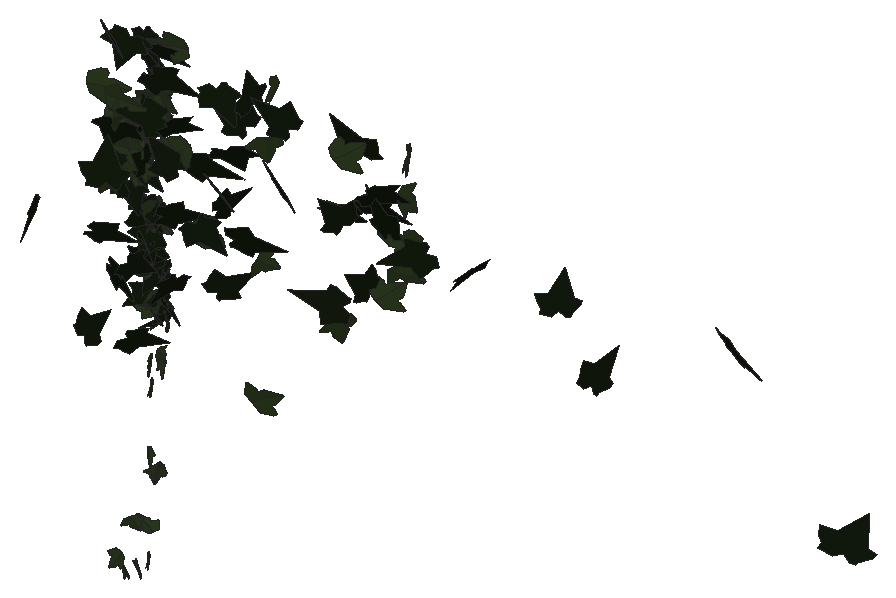
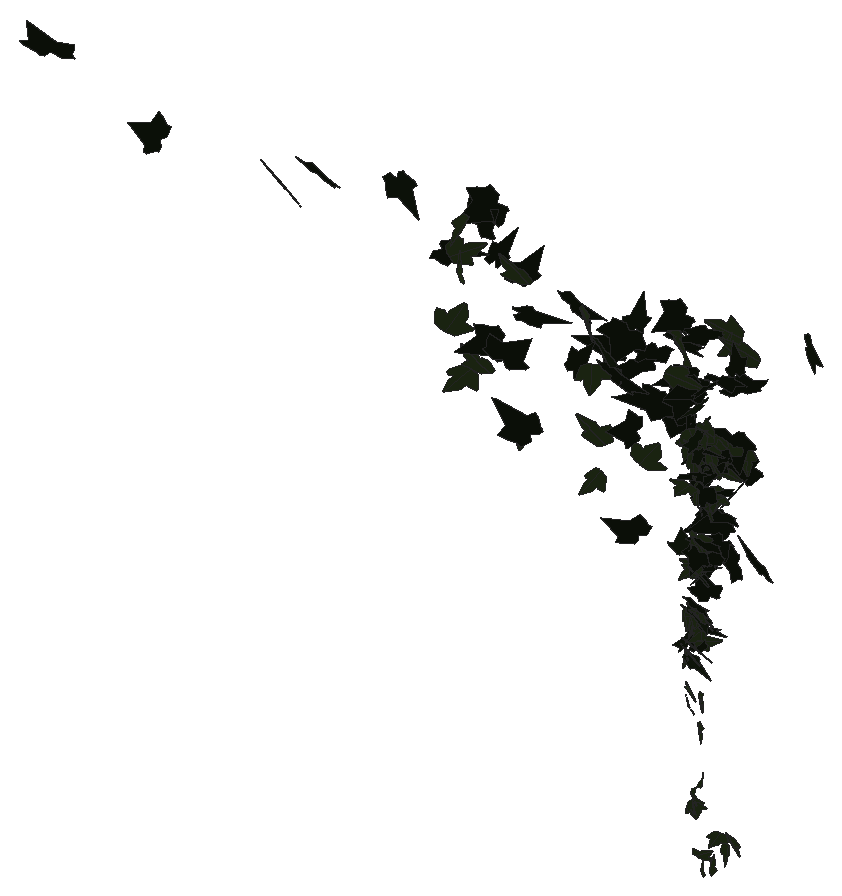
# SketchUp Ruby script. Lengths in inches.
U = 1.inch
M = Sketchup.active_model
def pt(a) = Geom::Point3d.new(a.map { |v| v * U })
def face(e, loops, mat)
  f = e.add_face(loops[0].map { |a| pt(a) })
  loops[1..].each { |l| e.add_face(l.map { |a| pt(a) }).erase! }
  f.material = f.back_material = mat if mat
  f
end
# faces: each face lists its corners as indices into pts; further lists are holes
def faces(e, pts, list, mat = nil) = list.each { |f| face(e, (f[0].is_a?(Array) ? f : [f]).map { |l| l.map { |i| pts[i] } }, mat) }
# xy, xz, yz: faces in a plane at the given z, y or x. An outline is a flat list of corners, or four numbers for a rectangle; further outlines are holes
def ring(l) = l.size == 4 ? [[l[0], l[1]], [l[2], l[1]], [l[2], l[3]], [l[0], l[3]]] : l.each_slice(2).to_a
def flat(e, list, mat, &to3) = list.each { |f| face(e, (f[0].is_a?(Array) ? f : [f]).map { |l| ring(l).map { |u, v| to3.(u, v) } }, mat) }
def xy(e, z, list, mat = nil) = flat(e, list, mat) { |x, y| [x, y, z] }
def xz(e, y, list, mat = nil) = flat(e, list, mat) { |x, z| [x, y, z] }
def yz(e, x, list, mat = nil) = flat(e, list, mat) { |y, z| [x, y, z] }
def lines(e, pts, list) = list.each { |a, b| e.add_line(pt(pts[a]), pt(pts[b])) }
# prism: a flat outline (further loops are holes) pulled along v
def prism(e, loops, v, mat = nil)
  f = face(e, loops, mat); d = Geom::Vector3d.new(v.map { |x| x * U })
  f.pushpull(f.normal.samedirection?(d) ? d.length : -d.length)
end
def box(e, o, s, mat = nil) = prism(e, [[o, [o[0] + s[0], o[1], o[2]], [o[0] + s[0], o[1] + s[1], o[2]], [o[0], o[1] + s[1], o[2]]]], [0, 0, s[2]], mat)
def at(x, y, z, deg = 0) = Geom::Transformation.translation(pt([x, y, z])) * Geom::Transformation.rotation(ORIGIN, Z_AXIS, deg.degrees)
def axes(o, x, y, z) = Geom::Transformation.new([*x, 0, *y, 0, *z, 0, *pt(o).to_a, 1])
def part(name) = M.definitions.add(name)
# library, detail: a bought-in or finely detailed component or shape, given as its bounding box
def library(name, o, s) = part(name).tap { |d| box(d.entities, o, s) }
def detail(e, o, s) = box(e.add_group.entities, o, s)
def put(e, d, t, mat = nil) = e.add_instance(d, t).tap { |i| i.material = mat if mat }
def group(e, t, mat = nil) = e.add_group.tap { |g| g.transformation = t; g.material = mat if mat }.entities
root = M.entities
M.materials.add("1026 AP 7946 SUNNY SIDE UP").color = [254, 231, 186]
M.materials.add("efeu1").color = [18, 25, 13]
M.materials.add("efeu2").color = [43, 57, 29]
c1 = part("ivyleaf_9")
p = [[1.54,2.16,1.25],[1.36,2.04,1.19],[-0.21,0.99,0.68],[-0.71,1.11,0.82],[-0.85,0.86,0.67],[-0.8,0.17,0.21],
  [-0.9,-0.01,0.1],[-0.67,-0.16,-0.02],[-0.08,-0.08,-0.05],[-0.03,-0.6,-0.4],[0.65,-0.88,-0.66],[0.83,-0.6,-0.49],
  [1.29,-0.42,-0.43],[1.8125,-0.07,-0.26],[1.21,0.44,0.15]]
faces(c1.entities,p,[[0,1,2,3,4,5,6,7,8,9,10,11,12,13,14]],"efeu1")
c2 = part("ivyleaf_10")
p = [[0,0.5,-0.03],[-0.0625,2.02,-0.43],[-0.19,2.01,-0.46],[-0.54,1.05,-0.29],[-0.52,0.625,-0.18],[-0.83,0.76,-0.28],
  [-1.16,0.64,-0.33],[-1.15,0.33,-0.24],[-0.77,-0.39,0.02],[-0.3,-0.51,0.16],[0.04,-0.48,0.23],[-0.02,2.01,-0.4375],
  [-0.06,2.01,-0.43],[0.04,-0.49,0.23],[0.67,-0.49,0.14],[1.38,0.36,-0.2],[1.375,0.51,-0.24],[0.81,0.65,-0.19],
  [0.62,0.59,-0.15],[0.6,1.09,-0.28],[0.5,1.23,-0.31]]
faces(c2.entities,p,[[0,1,2,3,4,5,6,7,8,9,10],[11,12,0,13,14,15,16,17,18,19,20]],"efeu2")
put(root,c1,axes([145.81,210.97,267.7],[-0.10226,-0.06705,0.33732],[0.10741,-0.32957,-0.05741],[0.51504,0.05542,0.07895]),"1026 AP 7946 SUNNY SIDE UP")
put(root,c2,axes([145.85,211.23,264.91],[0.40959,0.12772,-0.13372],[0.15878,0.08873,0.29755],[0.23926,-0.27752,0.03146]),"1026 AP 7946 SUNNY SIDE UP")
put(root,c2,axes([145.9375,211.7,251.53],[-0.19651,-0.13875,-0.10808],[0.14363,0.05646,-0.19013],[0.23189,-0.15255,0.02617]),"1026 AP 7946 SUNNY SIDE UP")
put(root,c1,axes([146.02,211.48,267.62],[-0.40394,-0.18707,-0.07784],[0.12417,0.01748,-0.32567],[0.29125,-0.2669,0.03089]),"1026 AP 7946 SUNNY SIDE UP")
put(root,c2,axes([146.15,212.33,251.04],[0.20297,0.0955,0.12839],[-0.19011,-0.0414,0.16215],[0.15645,-0.1742,0.03047]),"1026 AP 7946 SUNNY SIDE UP")
put(root,c2,axes([145.93,211.33,264.74],[-0.2012,0.25885,-0.12828],[0.08265,-0.11455,-0.29812],[-0.44507,-0.13829,0.00263]),"1026 AP 7946 SUNNY SIDE UP")
put(root,c2,axes([146.16,212.125,263.7],[-0.29001,-0.20187,0.08916],[-0.07666,-0.07409,-0.2818],[0.33749,-0.19031,0.01261]),"1026 AP 7946 SUNNY SIDE UP")
put(root,c2,axes([146.06,212.47,255.6875],[0.11639,-0.22167,-0.06838],[0.0122,0.07073,-0.23852],[0.36308,0.06868,0.02994]),"1026 AP 7946 SUNNY SIDE UP")
put(root,c1,axes([146.16,210.73,265.14],[0.34508,0.18415,-0.24138],[-0.24927,-0.17578,-0.29501],[-0.39831,0.26955,-0.0245]),"1026 AP 7946 SUNNY SIDE UP")
put(root,c1,axes([146.24,212.32,259.63],[-0.00974,0.25184,0.10049],[-0.11375,0.09106,-0.25007],[-0.4083,-0.03138,0.06727]),"1026 AP 7946 SUNNY SIDE UP")
put(root,c2,axes([146.1,212.53,259.7],[-0.35282,0.07848,0.00293],[-0.01517,-0.02036,-0.24391],[-0.12252,-0.22347,0.02177]),"1026 AP 7946 SUNNY SIDE UP")
put(root,c1,axes([146.14,211.09,262.98],[0.05251,-0.30731,-0.04227],[0.07696,-0.03379,0.31492],[-0.48103,-0.03895,0.04577]),"1026 AP 7946 SUNNY SIDE UP")
put(root,c2,axes([146.36,212.11,258.46],[-0.07709,-0.03468,-0.25525],[-0.37568,-0.06776,0.05812],[-0.1157,0.24312,-0.01865]),"1026 AP 7946 SUNNY SIDE UP")
put(root,c1,axes([145.99,212.43,261.75],[-0.06164,-0.24192,0.10022],[0.00245,-0.09998,-0.25251],[0.41081,-0.0357,0.01654]),"1026 AP 7946 SUNNY SIDE UP")
put(root,c1,axes([146.27,212.13,258.95],[-0.35397,-0.09187,0.08629],[-0.0999,-0.06514,-0.24835],[0.16867,-0.23138,0.03399]),"1026 AP 7946 SUNNY SIDE UP")
put(root,c2,axes([146.28,211.89,263.28],[0.11779,-0.11836,-0.26964],[-0.19717,0.22912,-0.14273],[0.4053,0.14585,0.00893]),"1026 AP 7946 SUNNY SIDE UP")
put(root,c2,axes([146.47,211.17,264.22],[0.13088,-0.03505,-0.33312],[-0.48796,0.09069,-0.09194],[0.15208,0.32114,-0.00834]),"1026 AP 7946 SUNNY SIDE UP")
put(root,c2,axes([146.18,211.76,265.04],[-0.0151,-0.29421,-0.00994],[0.00696,0.00784,-0.30318],[0.46274,-0.00972,0.00424]),"1026 AP 7946 SUNNY SIDE UP")
put(root,c1,axes([146.1,212.47,261.8],[0.37145,0.02124,-0.11874],[-0.17629,-0.0355,-0.24343],[-0.05431,0.26049,-0.02193]),"1026 AP 7946 SUNNY SIDE UP")
put(root,c1,axes([145.97,211.9,261.23],[-0.02565,-0.03067,0.28127],[0.38159,0.12698,0.03036],[-0.20311,0.24244,0.02151]),"1026 AP 7946 SUNNY SIDE UP")
put(root,c1,axes([145.98,211.65,263.65],[-0.03308,-0.26621,-0.14639],[0.07427,0.13626,-0.27231],[0.46752,-0.04048,0.0329]),"1026 AP 7946 SUNNY SIDE UP")
put(root,c2,axes([146.125,212.34,256.61],[0.15836,-0.22215,0.0476],[0.08028,-0.02846,-0.24898],[0.34806,0.10764,0.03577]),"1026 AP 7946 SUNNY SIDE UP")
put(root,c2,axes([146.14,212.28,265.875],[-0.34523,0.18958,-0.04181],[0.03447,-0.03828,-0.29869],[-0.30325,-0.22017,0.01364]),"1026 AP 7946 SUNNY SIDE UP")
put(root,c2,axes([146.21,212.57,252.85],[-0.20183,-0.157,0.04092],[0.01719,-0.06006,-0.20392],[0.25441,-0.12049,0.04624]),"1026 AP 7946 SUNNY SIDE UP")
put(root,c1,axes([145.97,212.49,265.4375],[0.33064,-0.18142,-0.01898],[-0.03977,-0.00275,-0.28548],[0.2838,0.21097,-0.01789]),"1026 AP 7946 SUNNY SIDE UP")
put(root,c2,axes([146.21,212.48,259.74],[0.26669,0.12797,-0.11203],[-0.11548,-0.08361,-0.2184],[-0.23829,0.18374,-0.01954]),"1026 AP 7946 SUNNY SIDE UP")
put(root,c2,axes([146.26,210.68,250.87],[0.29654,-0.1606,-0.07067],[-0.09168,0.03584,-0.25476],[0.25825,0.19714,-0.0093]),"1026 AP 7946 SUNNY SIDE UP")
put(root,c2,axes([146.23,211.51,264.84],[0.026,-0.23926,0.21925],[0.04147,-0.21273,-0.24816],[0.50323,0.02989,0.00912]),"1026 AP 7946 SUNNY SIDE UP")
put(root,c1,axes([146.05,212.01,260.18],[0.41203,0.05303,0.03617],[-0.06902,0.04477,0.27039],[0.07201,-0.26052,0.0522]),"1026 AP 7946 SUNNY SIDE UP")
put(root,c2,axes([146.24,212.57,252.97],[-0.10343,-0.19468,0.04011],[0.03786,-0.04967,-0.20834],[0.31022,-0.05885,0.0388]),"1026 AP 7946 SUNNY SIDE UP")
put(root,c1,axes([146.22,211.56,264.72],[0.23555,0.27996,0.02759],[0.03856,0.01542,-0.32668],[-0.4403,0.15112,-0.01385]),"1026 AP 7946 SUNNY SIDE UP")
put(root,c1,axes([146.24,212.25,260.875],[-0.26603,0.20692,-0.00281],[0.01116,0.01084,0.27512],[0.32523,0.16888,-0.01174]),"1026 AP 7946 SUNNY SIDE UP")
put(root,c1,axes([146.09,212.63,260.08],[-0.21443,-0.07293,-0.20014],[0.31084,0.02342,-0.1522],[0.09717,-0.23586,0.04524]),"1026 AP 7946 SUNNY SIDE UP")
put(root,c2,axes([146.24,211.59,263.54],[-0.13151,-0.30108,0.04679],[0.07258,-0.06083,-0.31626],[0.47365,-0.07427,0.06145]),"1026 AP 7946 SUNNY SIDE UP")
put(root,c1,axes([145.97,212.29,263.66],[-0.06827,-0.05391,0.27885],[0.29211,-0.20874,-0.01334],[0.32157,0.17817,0.07132]),"1026 AP 7946 SUNNY SIDE UP")
put(root,c1,axes([146.26,212.7,264.64],[-0.27548,-0.20601,0.02906],[-0.00375,-0.03641,-0.27792],[0.32719,-0.17387,0.02128]),"1026 AP 7946 SUNNY SIDE UP")
put(root,c1,axes([146.4375,212.47,258.01],[-0.23352,0.1948,-0.06346],[-0.01165,-0.08255,-0.24658],[-0.32158,-0.13847,0.05502]),"1026 AP 7946 SUNNY SIDE UP")
put(root,c1,axes([146.05,211.46,262.83],[-0.23725,-0.14339,-0.22558],[0.33357,0.07952,-0.20453],[0.23925,-0.25305,0.06146]),"1026 AP 7946 SUNNY SIDE UP")
put(root,c2,axes([146.09,212.5,263.61],[0.16217,-0.14058,0.21384],[0.22247,-0.15369,-0.17986],[0.32667,0.17445,0.01633]),"1026 AP 7946 SUNNY SIDE UP")
put(root,c2,axes([146.2,212.2,253.66],[-0.04298,0.20191,-0.10179],[0.00806,-0.10011,-0.21034],[-0.35416,-0.02678,0.00756]),"1026 AP 7946 SUNNY SIDE UP")
put(root,c1,axes([146.29,212.375,259.54],[-0.35994,-0.03623,-0.10592],[0.16742,-0.02522,-0.23567],[0.03533,-0.24958,0.03769]),"1026 AP 7946 SUNNY SIDE UP")
put(root,c1,axes([146.51,212.53,258.57],[-0.33225,0.12136,0.05052],[-0.07858,0.00986,-0.25043],[-0.18979,-0.21654,0.01524]),"1026 AP 7946 SUNNY SIDE UP")
put(root,c1,axes([146.1,212.1,267.53],[0.09089,-0.27667,-0.0949],[-0.02992,0.08853,-0.29065],[0.45676,0.06085,-0.00016]),"1026 AP 7946 SUNNY SIDE UP")
put(root,c1,axes([146.13,211.97,263.15],[0.12962,-0.1777,-0.21915],[-0.09651,0.20364,-0.19952],[0.42377,0.10073,0.02159]),"1026 AP 7946 SUNNY SIDE UP")
put(root,c2,axes([146.35,210.8,250.53],[-0.25275,0.17417,0.09181],[-0.11619,0.05137,-0.24314],[-0.28409,-0.17597,0.01776]),"1026 AP 7946 SUNNY SIDE UP")
put(root,c2,axes([146.32,212.46,265.06],[-0.0516,-0.27743,-0.06899],[0.01177,0.06496,-0.28742],[0.44803,-0.03366,-0.00039]),"1026 AP 7946 SUNNY SIDE UP")
put(root,c1,axes([146.05,212.61,265.85],[0.23516,-0.22985,0.06593],[0.03983,-0.06136,-0.2826],[0.37361,0.15122,-0.01137]),"1026 AP 7946 SUNNY SIDE UP")
put(root,c2,axes([146.16,211.87,263.57],[-0.24678,0.14556,-0.20685],[0.17209,-0.17365,-0.21794],[-0.3511,-0.18742,0.03857]),"1026 AP 7946 SUNNY SIDE UP")
put(root,c1,axes([146.15,212.13,262.02],[-0.19804,-0.16689,-0.18795],[0.24204,0.10599,-0.20982],[0.30286,-0.19383,0.04478]),"1026 AP 7946 SUNNY SIDE UP")
put(root,c1,axes([146.66,212.26,265.36],[-0.35967,0.03645,0.17002],[-0.26427,-0.02314,-0.23514],[-0.02489,-0.28099,0.03974]),"1026 AP 7946 SUNNY SIDE UP")
put(root,c1,axes([146.59,212.46,259.67],[-0.35192,0.1245,0.05876],[-0.09277,0.00947,-0.26298],[-0.19381,-0.23059,0.01918]),"1026 AP 7946 SUNNY SIDE UP")
put(root,c1,axes([146.25,211.4,265.03],[0.41211,0.1914,-0.04475],[-0.02803,-0.05076,-0.33318],[-0.30772,0.26096,-0.02958]),"1026 AP 7946 SUNNY SIDE UP")
put(root,c2,axes([146.29,211.7,264.65],[0.39612,-0.18235,0.06406],[0.06177,-0.05333,-0.32005],[0.29712,0.2542,-0.01887]),"1026 AP 7946 SUNNY SIDE UP")
put(root,c2,axes([146.42,212.09,261.99],[-0.11609,-0.27339,0.05903],[-0.01318,-0.05868,-0.29199],[0.43953,-0.07397,0.00683]),"1026 AP 7946 SUNNY SIDE UP")
put(root,c2,axes([146.49,212.33,259.24],[-0.11827,0.1245,0.22924],[-0.20099,0.18148,-0.14853],[-0.34579,-0.14807,0.00793]),"1026 AP 7946 SUNNY SIDE UP")
put(root,c2,axes([146.27,211.58,263.42],[0.48334,0.06936,0.02819],[0.04201,0.00414,-0.3246],[-0.10922,0.30854,-0.00008]),"1026 AP 7946 SUNNY SIDE UP")
put(root,c2,axes([146.38,211.72,263.98],[0.14656,0.28126,-0.10943],[0.03322,0.10648,0.30559],[0.47247,-0.09473,0.01246]),"1026 AP 7946 SUNNY SIDE UP")
put(root,c2,axes([146.57,209.64,264.07],[-0.48328,0.14747,0.14023],[-0.21714,0.02315,-0.34908],[-0.22774,-0.33501,0.03526]),"1026 AP 7946 SUNNY SIDE UP")
put(root,c1,axes([146.39,212.05,261.01],[-0.25678,-0.23255,0.00781],[0.01218,-0.0163,-0.29239],[0.36573,-0.16273,0.01522]),"1026 AP 7946 SUNNY SIDE UP")
put(root,c2,axes([146.41,211.45,250.0625],[-0.22915,0.16923,0.02664],[0.03898,-0.01147,0.22972],[0.26612,0.1474,-0.0107]),"1026 AP 7946 SUNNY SIDE UP")
put(root,c2,axes([146.35,212.14,261.05],[0.0436,-0.11907,0.26217],[-0.01753,0.25573,0.12568],[-0.4424,-0.02187,0.02086]),"1026 AP 7946 SUNNY SIDE UP")
put(root,c1,axes([146.375,212.18,258.24],[0.25028,-0.18952,0.0388],[-0.01078,0.04461,0.25411],[-0.30397,-0.15763,0.02294]),"1026 AP 7946 SUNNY SIDE UP")
put(root,c1,axes([146.24,212.12,260.83],[0.0475,-0.26812,0.0869],[0.00268,-0.08619,-0.27836],[0.44268,0.02929,-0.00764]),"1026 AP 7946 SUNNY SIDE UP")
put(root,c2,axes([146.36,212.41,253.13],[0.14963,-0.16183,0.11258],[0.08655,-0.09548,-0.19396],[0.29544,0.10993,-0.0002]),"1026 AP 7946 SUNNY SIDE UP")
put(root,c2,axes([146.32,212.09,258.8],[-0.07345,-0.12106,-0.22947],[0.18039,0.19111,-0.13108],[0.35442,-0.12236,0.01916]),"1026 AP 7946 SUNNY SIDE UP")
put(root,c2,axes([146.27,212.41,261.18],[0.09609,0.17105,0.19688],[0.11026,0.17679,-0.18603],[-0.38673,0.0929,-0.00412]),"1026 AP 7946 SUNNY SIDE UP")
put(root,c2,axes([146.25,212.6,256.77],[-0.0221,-0.11135,-0.19889],[0.16471,-0.17338,0.09447],[-0.30834,-0.08464,0.06472]),"1026 AP 7946 SUNNY SIDE UP")
put(root,c2,axes([146.2,212.22,261.36],[0.08786,0.01851,-0.27095],[0.31203,0.17423,0.05706],[0.27323,-0.20493,0.02197]),"1026 AP 7946 SUNNY SIDE UP")
put(root,c2,axes([146.42,212.34,264.99],[0.29779,-0.19947,0.04295],[0.02432,-0.04422,-0.28294],[0.31987,0.18906,-0.01847]),"1026 AP 7946 SUNNY SIDE UP")
put(root,c1,axes([146.54,212.57,258.32],[-0.3351,0.05751,-0.12114],[0.16403,-0.06211,-0.2258],[-0.12509,-0.2355,0.02842]),"1026 AP 7946 SUNNY SIDE UP")
put(root,c2,axes([146.34,212.65,256.45],[0.18315,-0.08784,0.17109],[0.17459,-0.12616,-0.14926],[0.23917,0.15937,-0.02206]),"1026 AP 7946 SUNNY SIDE UP")
put(root,c2,axes([146.22,211.52,265.45],[0.41283,0.11181,0.16867],[0.25911,0.02614,-0.29158],[-0.17187,0.30797,-0.03444]),"1026 AP 7946 SUNNY SIDE UP")
put(root,c1,axes([146.28,212.11,266.83],[0.29721,-0.19278,-0.11771],[-0.04929,0.12387,-0.27061],[0.34803,0.18218,0.0622]),"1026 AP 7946 SUNNY SIDE UP")
put(root,c2,axes([146.59,212.25,265.76],[-0.2532,-0.23164,0.04363],[-0.01861,-0.04487,-0.29044],[0.37018,-0.1607,0.01524]),"1026 AP 7946 SUNNY SIDE UP")
put(root,c2,axes([146.39,211.92,250.29],[0.0365,-0.03699,0.20445],[0.19351,-0.15603,-0.04565],[0.25204,0.12515,0.00544]),"1026 AP 7946 SUNNY SIDE UP")
put(root,c2,axes([146.56,212.14,262.03],[0.20287,-0.2582,-0.01842],[-0.03671,0.00665,-0.29675],[0.40516,0.12989,-0.01766]),"1026 AP 7946 SUNNY SIDE UP")
put(root,c2,axes([146.6,212.47,259.54],[0.02387,-0.2516,-0.07013],[0.01757,0.06733,-0.25883],[0.40888,0.01179,0.01522]),"1026 AP 7946 SUNNY SIDE UP")
put(root,c2,axes([146.54,212.61,257.83],[-0.16848,0.16377,0.15205],[0.1515,-0.11166,0.20032],[0.31071,0.14325,-0.01523]),"1026 AP 7946 SUNNY SIDE UP")
put(root,c1,axes([146.23,210.44,260.52],[0.08487,-0.03552,-0.37789],[0.57497,-0.03932,0.05915],[-0.06953,-0.36847,0.02792]),"1026 AP 7946 SUNNY SIDE UP")
put(root,c2,axes([146.65,212.2,265.38],[-0.43733,0.05726,-0.02744],[0.03243,-0.03285,-0.29131],[-0.09408,-0.27749,0.02711]),"1026 AP 7946 SUNNY SIDE UP")
put(root,c2,axes([146.32,211.64,265.6],[0.02003,-0.01534,0.30949],[0.46822,-0.04261,-0.01549],[0.06803,0.29775,0.01551]),"1026 AP 7946 SUNNY SIDE UP")
put(root,c1,axes([146.47,212.58,258.61],[0.1926,-0.21027,0.04686],[0.02195,-0.04583,-0.25071],[0.33797,0.12281,-0.01042]),"1026 AP 7946 SUNNY SIDE UP")
put(root,c1,axes([146.68,211.39,263.71],[0.03063,0.06479,0.36075],[-0.25628,-0.30978,0.06665],[0.49724,-0.16365,0.01213]),"1026 AP 7946 SUNNY SIDE UP")
put(root,c2,axes([146.64,212.33,263.93],[0.31344,0.1117,0.1549],[0.21379,0.0634,-0.23483],[-0.20142,0.24111,-0.0082]),"1026 AP 7946 SUNNY SIDE UP")
put(root,c1,axes([146.6875,208.64,259.3],[-0.18536,0.26211,0.27056],[0.20143,-0.2282,0.29421],[0.54579,0.17324,-0.0167]),"1026 AP 7946 SUNNY SIDE UP")
put(root,c1,axes([146.63,211.93,267.25],[0.43231,0.06873,0.10567],[0.162,0.00856,-0.29145],[-0.10608,0.29319,-0.01445]),"1026 AP 7946 SUNNY SIDE UP")
put(root,c2,axes([147.38,212.1,267.5],[0.11678,-0.00743,-0.36427],[-0.55169,0.04362,-0.07662],[0.06952,0.35863,0.00391]),"1026 AP 7946 SUNNY SIDE UP")
put(root,c1,axes([146.79,211.62,265.65],[0.07073,-0.31806,0.0566],[0.00235,-0.05709,-0.33119],[0.50802,0.04454,-0.00635]),"1026 AP 7946 SUNNY SIDE UP")
put(root,c1,axes([146.93,210.34,260.97],[0.00055,0.00298,-0.38455],[-0.18987,0.35322,0.00486],[0.55543,0.12075,0.00204]),"1026 AP 7946 SUNNY SIDE UP")
put(root,c1,axes([146.82,212.22,261.5],[-0.17936,-0.25739,0.02893],[0.40235,-0.11698,-0.03283],[0.06381,0.01414,0.28833]),"1026 AP 7946 SUNNY SIDE UP")
put(root,c2,axes([146.55,209.33,267.23],[0.1653,-0.07761,-0.39266],[0.58947,-0.08338,0.12366],[-0.16053,-0.38606,0.04977]),"1026 AP 7946 SUNNY SIDE UP")
put(root,c1,axes([147.26,211.41,265.75],[0.15913,-0.04388,-0.34466],[-0.50299,0.09785,-0.11242],[0.16761,0.33531,-0.01014]),"1026 AP 7946 SUNNY SIDE UP")
put(root,c1,axes([147.07,208.64,262.83],[0.40977,0.11138,0.23082],[0.34911,0.04427,-0.28926],[-0.17948,0.3404,-0.03566]),"1026 AP 7946 SUNNY SIDE UP")
put(root,c1,axes([147.56,205.23,265.42],[-0.3099,0.09978,-0.34649],[0.42499,-0.20378,-0.22626],[-0.35305,-0.3329,0.03179]),"1026 AP 7946 SUNNY SIDE UP")
put(root,c1,axes([147.32,211.09,267],[0.06101,0.0023,-0.37742],[0.2679,0.32605,0.0226],[0.51001,-0.17154,0.03328]),"1026 AP 7946 SUNNY SIDE UP")
put(root,c1,axes([147.86,208.12,265.04],[-0.43759,-0.14871,0.27973],[0.33836,0.17113,0.32376],[-0.35158,0.34978,-0.03657]),"1026 AP 7946 SUNNY SIDE UP")
put(root,c2,axes([147.87,208.57,266.99],[-0.00046,-0.06205,-0.39859],[0.09405,0.38201,-0.06099],[0.60838,-0.0591,0.00913]),"1026 AP 7946 SUNNY SIDE UP")
put(root,c2,axes([147.625,208.75,267.39],[-0.07193,-0.00113,0.38597],[0.58102,0.06224,0.04704],[-0.09737,0.37228,-0.00445]),"1026 AP 7946 SUNNY SIDE UP")
put(root,c2,axes([148.03,210.4,266.71],[0.29166,-0.07409,0.32468],[0.42623,-0.16396,-0.20474],[0.27954,0.32729,-0.02658]),"1026 AP 7946 SUNNY SIDE UP")
put(root,c1,axes([149.04,209.13,267.07],[-0.16789,-0.23438,-0.2851],[-0.17001,-0.25334,0.26381],[-0.54264,0.15189,0.00556]),"1026 AP 7946 SUNNY SIDE UP")
put(root,c1,axes([148.76,208.0625,260.11],[0.00382,0.12461,-0.35379],[0.02938,0.34364,0.13034],[0.57474,-0.0184,-0.00431]),"1026 AP 7946 SUNNY SIDE UP")
put(root,c1,axes([149.29,211.5,267],[-0.05361,-0.28963,-0.22642],[0.03281,0.21717,-0.29914],[0.56919,-0.0398,-0.00408]),"1026 AP 7946 SUNNY SIDE UP")
put(root,c1,axes([149.32,210.35,265.14],[0.1701,0.08759,-0.36038],[0.33974,0.27731,0.14179],[0.45494,-0.23984,0.02886]),"1026 AP 7946 SUNNY SIDE UP")
put(root,c1,axes([150.25,211.5,266.22],[-0.17544,0.17112,0.37707],[-0.41973,0.2525,-0.20451],[-0.47508,-0.28627,0.04144]),"1026 AP 7946 SUNNY SIDE UP")
put(root,c1,axes([150.17,208.45,266.12],[-0.50906,-0.04824,-0.15994],[-0.24851,0.01498,0.33542],[-0.0581,0.35861,-0.03338]),"1026 AP 7946 SUNNY SIDE UP")
put(root,c2,axes([150.04,210.25,262.78],[-0.50375,-0.00849,-0.18122],[-0.27671,0.02681,0.32909],[0.00862,0.36448,-0.02628]),"1026 AP 7946 SUNNY SIDE UP")
put(root,c1,axes([149.54,208.75,264.13],[0.2755,0.12638,0.33216],[0.46802,0.1282,-0.21813],[-0.27629,0.34316,-0.03828]),"1026 AP 7946 SUNNY SIDE UP")
put(root,c1,axes([149.64,211.125,260.67],[-0.05109,0.01179,0.37311],[0.5339,0.1278,0.02785],[-0.1987,0.34036,-0.02111]),"1026 AP 7946 SUNNY SIDE UP")
put(root,c1,axes([149.81,208.6,267.26],[0.29609,0.2254,0.21754],[0.25021,0.13943,-0.30052],[-0.41464,0.24509,-0.026]),"1026 AP 7946 SUNNY SIDE UP")
put(root,c2,axes([150.28,208.67,266.6875],[0.43157,-0.22903,-0.16364],[-0.21236,0.08365,-0.36718],[0.38205,0.30521,-0.01924]),"1026 AP 7946 SUNNY SIDE UP")
put(root,c1,axes([150.51,211.5625,267.02],[-0.44002,0.15458,-0.28158],[-0.35444,0.15769,0.32949],[0.34548,0.35866,-0.02061]),"1026 AP 7946 SUNNY SIDE UP")
put(root,c1,axes([150.19,210.49,263.84],[0.05598,0.09354,0.38414],[0.3828,0.28365,-0.09573],[-0.46678,0.24383,-0.03244]),"1026 AP 7946 SUNNY SIDE UP")
put(root,c1,axes([150.78,207.67,262.92],[-0.11744,0.21466,-0.3],[0.09795,-0.28653,-0.23476],[-0.56192,-0.09481,0.02178]),"1026 AP 7946 SUNNY SIDE UP")
put(root,c2,axes([151.19,211.4,266.03],[-0.31877,-0.30671,-0.0375],[0.06275,0.01507,-0.3778],[0.48127,-0.20512,0.02442]),"1026 AP 7946 SUNNY SIDE UP")
put(root,c2,axes([151.17,211.14,262.18],[-0.11869,-0.20754,-0.30542],[0.21537,0.26264,-0.2247],[0.52507,-0.15464,0.02313]),"1026 AP 7946 SUNNY SIDE UP")
put(root,c1,axes([151.25,209.53,266.55],[0.41842,0.27035,-0.0276],[-0.00451,-0.03684,-0.39025],[-0.4274,0.26506,-0.0229]),"1026 AP 7946 SUNNY SIDE UP")
put(root,c2,axes([151.45,211.44,267.94],[0.23093,-0.32676,-0.0991],[-0.0821,0.07988,-0.3683],[0.52844,0.15521,-0.01392]),"1026 AP 7946 SUNNY SIDE UP")
put(root,c1,axes([151.59,207.71,265.02],[0.02855,-0.19197,-0.3301],[-0.0081,0.31955,-0.19633],[0.58581,0.01377,0.01338]),"1026 AP 7946 SUNNY SIDE UP")
put(root,c1,axes([151.93,208.27,265.96],[0.41665,-0.2601,-0.05868],[0.09258,-0.01901,0.38136],[-0.4078,-0.27005,0.02662]),"1026 AP 7946 SUNNY SIDE UP")
put(root,c1,axes([152.67,210.48,267.42],[-0.15714,0.13776,0.36286],[-0.40163,0.243,-0.17153],[-0.43702,-0.27286,0.02717]),"1026 AP 7946 SUNNY SIDE UP")
put(root,c1,axes([152.67,210.39,265.14],[0.20065,-0.30566,0.21643],[-0.10651,0.2011,0.34215],[-0.57497,-0.14392,0.01215]),"1026 AP 7946 SUNNY SIDE UP")
put(root,c1,axes([152.82,212.5,263.77],[0.52379,0.18519,-0.09315],[0.09764,0.07576,0.39142],[0.30975,-0.33704,0.03413]),"1026 AP 7946 SUNNY SIDE UP")
put(root,c1,axes([152.77,208.06,264.77],[0.29111,0.00429,0.32885],[0.49354,-0.06966,-0.18699],[0.09144,0.36236,-0.03764]),"1026 AP 7946 SUNNY SIDE UP")
put(root,c1,axes([153.75,212.53,266.07],[0.25993,-0.05347,0.36424],[-0.48493,0.17648,0.17692],[-0.28551,-0.34843,0.03111]),"1026 AP 7946 SUNNY SIDE UP")
put(root,c2,axes([154.43,206.92,260.53],[-0.40064,-0.0143,0.28974],[0.43231,0.06997,0.26059],[-0.09643,0.37306,-0.03551]),"1026 AP 7946 SUNNY SIDE UP")
put(root,c2,axes([155.16,209.88,262.11],[-0.23918,-0.36085,-0.07136],[0.06315,0.05596,-0.4028],[0.5737,-0.1566,0.01458]),"1026 AP 7946 SUNNY SIDE UP")
put(root,c2,axes([154.97,210.12,267.42],[0.46097,-0.10239,-0.24959],[0.38223,-0.03081,0.31702],[-0.15573,-0.3787,0.0393]),"1026 AP 7946 SUNNY SIDE UP")
put(root,c1,axes([155.12,211.08,265.52],[0.52951,0.07025,0.16757],[0.2611,-0.00573,-0.3525],[-0.09552,0.37376,-0.03463]),"1026 AP 7946 SUNNY SIDE UP")
put(root,c1,axes([156.21,208.59,266.32],[0.12257,0.13151,0.3797],[-0.48064,-0.213,0.14394],[0.38243,-0.30984,0.05921]),"1026 AP 7946 SUNNY SIDE UP")
put(root,c1,axes([157.01,207.52,264.3],[-0.29597,-0.18296,-0.28469],[-0.32919,-0.17919,0.26909],[-0.40224,0.28127,-0.01075]),"1026 AP 7946 SUNNY SIDE UP")
put(root,c2,axes([156.49,210.99,263.87],[-0.28199,-0.20643,-0.27838],[0.31013,0.18409,-0.27987],[0.43377,-0.26582,0.01913]),"1026 AP 7946 SUNNY SIDE UP")
put(root,c2,axes([156.61,211.16,267.59],[0.09635,-0.06319,0.38477],[0.35521,-0.29806,-0.09179],[0.47881,0.23383,-0.00933]),"1026 AP 7946 SUNNY SIDE UP")
put(root,c2,axes([156.72,209.84,263.52],[0.4728,-0.06276,-0.23838],[0.36776,-0.0022,0.31419],[-0.08039,-0.37919,0.03535]),"1026 AP 7946 SUNNY SIDE UP")
put(root,c2,axes([157.85,210.09,264.73],[-0.40919,-0.21952,-0.21896],[-0.28454,-0.11221,0.34904],[-0.38545,0.31588,-0.02521]),"1026 AP 7946 SUNNY SIDE UP")
put(root,c1,axes([157.79,207.93,268.1],[0.40159,0.25353,0.22728],[0.28712,0.12581,-0.36838],[-0.44189,0.31216,-0.0328]),"1026 AP 7946 SUNNY SIDE UP")
put(root,c1,axes([158.45,207.91,267.14],[0.17079,-0.11422,0.40451],[-0.27446,0.35519,0.158],[-0.58257,-0.20082,0.04415]),"1026 AP 7946 SUNNY SIDE UP")
put(root,c2,axes([158.24,208.92,267.74],[-0.07342,0.29696,0.27504],[-0.10329,0.25771,-0.30759],[-0.61757,-0.07841,0.01874]),"1026 AP 7946 SUNNY SIDE UP")
put(root,c1,axes([158.41,207.08,265.56],[0.04181,0.0661,0.39721],[-0.39098,-0.295,0.06811],[0.47411,-0.2491,0.02114]),"1026 AP 7946 SUNNY SIDE UP")
put(root,c2,axes([158.65,208.74,266.41],[-0.15396,-0.11623,-0.36904],[-0.46356,-0.20558,0.15081],[-0.36691,0.30851,-0.03567]),"1026 AP 7946 SUNNY SIDE UP")
put(root,c1,axes([159.2,208.64,266.3125],[-0.06998,-0.12744,-0.37776],[-0.06865,-0.36438,0.13405],[-0.60546,0.05605,0.02846]),"1026 AP 7946 SUNNY SIDE UP")
put(root,c1,axes([161.97,207.49,267.28],[-0.16137,0.35643,-0.15967],[0.05141,-0.15392,-0.38286],[-0.61026,-0.10721,0.00997]),"1026 AP 7946 SUNNY SIDE UP")
put(root,c1,axes([164.75,207.99,266.75],[-0.56418,0.18756,0.01314],[0.04168,0.02557,0.41569],[0.29254,0.35808,-0.03388]),"1026 AP 7946 SUNNY SIDE UP")
put(root,c1,axes([166.59,207.25,265.23],[-0.35685,0.36274,0.13799],[0.12791,-0.10461,0.43999],[0.59327,0.24074,-0.01186]),"1026 AP 7946 SUNNY SIDE UP")
put(root,c1,axes([169.95,209.33,266.76],[0.31753,-0.26301,0.29549],[0.24084,-0.24518,-0.34235],[0.56441,0.25258,-0.02016]),"1026 AP 7946 SUNNY SIDE UP")
put(root,c1,axes([178.08,204.53,264.89],[-0.478,0.073,0.3192],[0.48177,-0.04701,0.32125],[0.13344,0.43122,-0.01639]),"1026 AP 7946 SUNNY SIDE UP")
